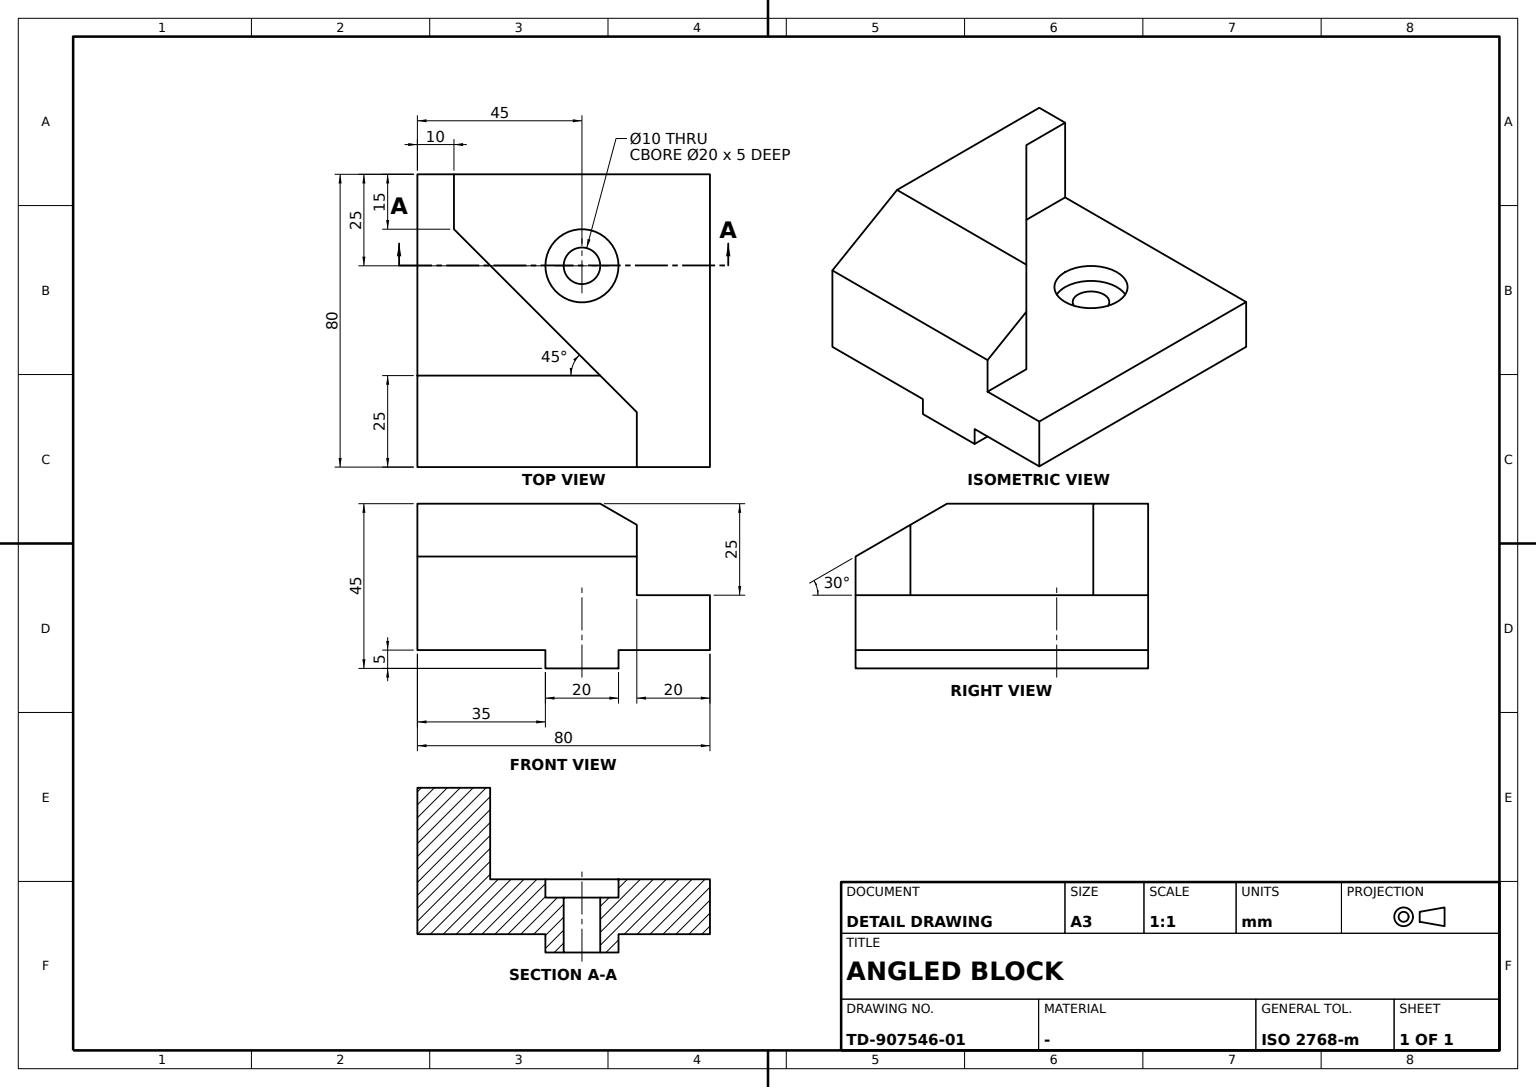
ISO-10303-21;
HEADER;
FILE_DESCRIPTION((''),'2;1');
FILE_NAME('','',(''),(''),'','','');
FILE_SCHEMA(('AUTOMOTIVE_DESIGN'));
ENDSEC;
DATA;
#1=APPLICATION_CONTEXT('');
#2=PRODUCT_CONTEXT('',#1,'mechanical');
#3=PRODUCT('','','',(#2));
#4=PRODUCT_DEFINITION_FORMATION('','',#3);
#5=PRODUCT_DEFINITION_CONTEXT('',#1,'design');
#6=PRODUCT_DEFINITION('','',#4,#5);
#7=PRODUCT_DEFINITION_SHAPE('','',#6);
#8=(LENGTH_UNIT()NAMED_UNIT(*)SI_UNIT(.MILLI.,.METRE.));
#9=(NAMED_UNIT(*)PLANE_ANGLE_UNIT()SI_UNIT($,.RADIAN.));
#10=(NAMED_UNIT(*)SI_UNIT($,.STERADIAN.)SOLID_ANGLE_UNIT());
#11=UNCERTAINTY_MEASURE_WITH_UNIT(LENGTH_MEASURE(0.005),#8,'distance_accuracy_value','');
#12=(GEOMETRIC_REPRESENTATION_CONTEXT(3)GLOBAL_UNCERTAINTY_ASSIGNED_CONTEXT((#11))GLOBAL_UNIT_ASSIGNED_CONTEXT((#8,#9,#10))REPRESENTATION_CONTEXT('',''));
#13=CARTESIAN_POINT('',(50.,15.,-5.));
#14=VERTEX_POINT('',#13);
#15=CARTESIAN_POINT('',(45.,15.,-5.));
#16=DIRECTION('',(0.,0.,1.));
#17=DIRECTION('',(1.,0.,0.));
#18=AXIS2_PLACEMENT_3D('',#15,#16,#17);
#19=CIRCLE('',#18,5.);
#20=EDGE_CURVE('',#14,#14,#19,.T.);
#21=ORIENTED_EDGE('',*,*,#20,.F.);
#22=EDGE_LOOP('',(#21));
#23=FACE_BOUND('',#22,.T.);
#24=CARTESIAN_POINT('',(40.,15.,10.));
#25=VERTEX_POINT('',#24);
#26=CARTESIAN_POINT('',(45.,15.,10.));
#27=DIRECTION('',(0.,0.,-1.));
#28=DIRECTION('',(-1.,0.,0.));
#29=AXIS2_PLACEMENT_3D('',#26,#27,#28);
#30=CIRCLE('',#29,5.);
#31=EDGE_CURVE('',#25,#25,#30,.T.);
#32=ORIENTED_EDGE('',*,*,#31,.F.);
#33=EDGE_LOOP('',(#32));
#34=FACE_BOUND('',#33,.T.);
#35=CARTESIAN_POINT('',(45.,15.,9.9));
#36=AXIS2_PLACEMENT_3D('',#35,#27,#17);
#37=CYLINDRICAL_SURFACE('',#36,5.);
#38=ADVANCED_FACE('',(#23,#34),#37,.F.);
#39=CARTESIAN_POINT('',(55.,40.,0.));
#40=VERTEX_POINT('',#39);
#41=CARTESIAN_POINT('',(55.,-40.,0.));
#42=VERTEX_POINT('',#41);
#43=CARTESIAN_POINT('',(55.,0.,0.));
#44=DIRECTION('',(0.,-1.,0.));
#45=VECTOR('',#44,1000.);
#46=LINE('',#43,#45);
#47=EDGE_CURVE('',#40,#42,#46,.T.);
#48=ORIENTED_EDGE('',*,*,#47,.F.);
#49=CARTESIAN_POINT('',(80.,40.,0.));
#50=VERTEX_POINT('',#49);
#51=VECTOR('',#28,1000.);
#52=LINE('',#49,#51);
#53=EDGE_CURVE('',#50,#40,#52,.T.);
#54=ORIENTED_EDGE('',*,*,#53,.F.);
#55=CARTESIAN_POINT('',(80.,-40.,0.));
#56=VERTEX_POINT('',#55);
#57=CARTESIAN_POINT('',(80.,0.,0.));
#58=LINE('',#57,#45);
#59=EDGE_CURVE('',#50,#56,#58,.T.);
#60=ORIENTED_EDGE('',*,*,#59,.T.);
#61=LINE('',#55,#51);
#62=EDGE_CURVE('',#56,#42,#61,.T.);
#63=ORIENTED_EDGE('',*,*,#62,.T.);
#64=EDGE_LOOP('',(#48,#54,#60,#63));
#65=FACE_BOUND('',#64,.T.);
#66=AXIS2_PLACEMENT_3D('',#57,#16,#28);
#67=PLANE('',#66);
#68=ADVANCED_FACE('',(#65),#67,.F.);
#69=CARTESIAN_POINT('',(60.,-40.,25.566243));
#70=VERTEX_POINT('',#69);
#71=CARTESIAN_POINT('',(60.,-25.,34.226497));
#72=VERTEX_POINT('',#71);
#73=DIRECTION('',(0.,0.866025404,0.5));
#74=VECTOR('',#73,1000.);
#75=LINE('',#69,#74);
#76=EDGE_CURVE('',#70,#72,#75,.T.);
#77=ORIENTED_EDGE('',*,*,#76,.T.);
#78=CARTESIAN_POINT('',(50.,-15.,40.));
#79=VERTEX_POINT('',#78);
#80=CARTESIAN_POINT('',(21.900181,13.099819,56.223438));
#81=DIRECTION('',(0.654653671,-0.654653671,-0.377964473));
#82=VECTOR('',#81,1000.);
#83=LINE('',#80,#82);
#84=EDGE_CURVE('',#79,#72,#83,.T.);
#85=ORIENTED_EDGE('',*,*,#84,.F.);
#86=CARTESIAN_POINT('',(0.,-15.,40.));
#87=VERTEX_POINT('',#86);
#88=VECTOR('',#17,1000.);
#89=LINE('',#86,#88);
#90=EDGE_CURVE('',#87,#79,#89,.T.);
#91=ORIENTED_EDGE('',*,*,#90,.F.);
#92=CARTESIAN_POINT('',(0.,-40.,25.566243));
#93=VERTEX_POINT('',#92);
#94=CARTESIAN_POINT('',(0.,-21.070508,36.495191));
#95=LINE('',#94,#74);
#96=EDGE_CURVE('',#93,#87,#95,.T.);
#97=ORIENTED_EDGE('',*,*,#96,.F.);
#98=LINE('',#92,#88);
#99=EDGE_CURVE('',#93,#70,#98,.T.);
#100=ORIENTED_EDGE('',*,*,#99,.T.);
#101=EDGE_LOOP('',(#77,#85,#91,#97,#100));
#102=FACE_BOUND('',#101,.T.);
#103=DIRECTION('',(0.,0.5,-0.866025404));
#104=AXIS2_PLACEMENT_3D('',#92,#103,#73);
#105=PLANE('',#104);
#106=ADVANCED_FACE('',(#102),#105,.F.);
#107=CARTESIAN_POINT('',(55.,40.,-5.));
#108=VERTEX_POINT('',#107);
#109=VECTOR('',#27,1000.);
#110=LINE('',#39,#109);
#111=EDGE_CURVE('',#40,#108,#110,.T.);
#112=ORIENTED_EDGE('',*,*,#111,.F.);
#113=ORIENTED_EDGE('',*,*,#47,.T.);
#114=CARTESIAN_POINT('',(55.,-40.,-5.));
#115=VERTEX_POINT('',#114);
#116=LINE('',#41,#109);
#117=EDGE_CURVE('',#42,#115,#116,.T.);
#118=ORIENTED_EDGE('',*,*,#117,.T.);
#119=CARTESIAN_POINT('',(55.,0.,-5.));
#120=LINE('',#119,#45);
#121=EDGE_CURVE('',#108,#115,#120,.T.);
#122=ORIENTED_EDGE('',*,*,#121,.F.);
#123=EDGE_LOOP('',(#112,#113,#118,#122));
#124=FACE_BOUND('',#123,.T.);
#125=AXIS2_PLACEMENT_3D('',#43,#28,#27);
#126=PLANE('',#125);
#127=ADVANCED_FACE('',(#124),#126,.F.);
#128=ORIENTED_EDGE('',*,*,#84,.T.);
#129=CARTESIAN_POINT('',(60.,-25.,15.));
#130=VERTEX_POINT('',#129);
#131=LINE('',#129,#109);
#132=EDGE_CURVE('',#72,#130,#131,.T.);
#133=ORIENTED_EDGE('',*,*,#132,.T.);
#134=CARTESIAN_POINT('',(10.,25.,15.));
#135=VERTEX_POINT('',#134);
#136=DIRECTION('',(0.707106781,-0.707106781,0.));
#137=VECTOR('',#136,1000.);
#138=LINE('',#134,#137);
#139=EDGE_CURVE('',#135,#130,#138,.T.);
#140=ORIENTED_EDGE('',*,*,#139,.F.);
#141=CARTESIAN_POINT('',(10.,25.,40.));
#142=VERTEX_POINT('',#141);
#143=VECTOR('',#16,1000.);
#144=LINE('',#141,#143);
#145=EDGE_CURVE('',#135,#142,#144,.T.);
#146=ORIENTED_EDGE('',*,*,#145,.T.);
#147=LINE('',#141,#137);
#148=EDGE_CURVE('',#142,#79,#147,.T.);
#149=ORIENTED_EDGE('',*,*,#148,.T.);
#150=EDGE_LOOP('',(#128,#133,#140,#146,#149));
#151=FACE_BOUND('',#150,.T.);
#152=DIRECTION('',(-0.707106781,-0.707106781,0.));
#153=AXIS2_PLACEMENT_3D('',#134,#152,#136);
#154=PLANE('',#153);
#155=ADVANCED_FACE('',(#151),#154,.F.);
#156=CARTESIAN_POINT('',(35.,40.,-5.));
#157=VERTEX_POINT('',#156);
#158=CARTESIAN_POINT('',(35.,40.,0.));
#159=VERTEX_POINT('',#158);
#160=LINE('',#156,#143);
#161=EDGE_CURVE('',#157,#159,#160,.T.);
#162=ORIENTED_EDGE('',*,*,#161,.T.);
#163=CARTESIAN_POINT('',(0.,40.,0.));
#164=VERTEX_POINT('',#163);
#165=EDGE_CURVE('',#159,#164,#52,.T.);
#166=ORIENTED_EDGE('',*,*,#165,.T.);
#167=CARTESIAN_POINT('',(0.,40.,40.));
#168=VERTEX_POINT('',#167);
#169=LINE('',#163,#143);
#170=EDGE_CURVE('',#164,#168,#169,.T.);
#171=ORIENTED_EDGE('',*,*,#170,.T.);
#172=CARTESIAN_POINT('',(10.,40.,40.));
#173=VERTEX_POINT('',#172);
#174=LINE('',#167,#88);
#175=EDGE_CURVE('',#168,#173,#174,.T.);
#176=ORIENTED_EDGE('',*,*,#175,.T.);
#177=CARTESIAN_POINT('',(10.,40.,15.));
#178=VERTEX_POINT('',#177);
#179=LINE('',#172,#109);
#180=EDGE_CURVE('',#173,#178,#179,.T.);
#181=ORIENTED_EDGE('',*,*,#180,.T.);
#182=CARTESIAN_POINT('',(80.,40.,15.));
#183=VERTEX_POINT('',#182);
#184=LINE('',#177,#88);
#185=EDGE_CURVE('',#178,#183,#184,.T.);
#186=ORIENTED_EDGE('',*,*,#185,.T.);
#187=LINE('',#182,#109);
#188=EDGE_CURVE('',#183,#50,#187,.T.);
#189=ORIENTED_EDGE('',*,*,#188,.T.);
#190=ORIENTED_EDGE('',*,*,#53,.T.);
#191=ORIENTED_EDGE('',*,*,#111,.T.);
#192=LINE('',#107,#51);
#193=EDGE_CURVE('',#108,#157,#192,.T.);
#194=ORIENTED_EDGE('',*,*,#193,.T.);
#195=EDGE_LOOP('',(#162,#166,#171,#176,#181,#186,#189,#190,#191,#194));
#196=FACE_BOUND('',#195,.T.);
#197=DIRECTION('',(0.,1.,0.));
#198=AXIS2_PLACEMENT_3D('',#163,#197,#28);
#199=PLANE('',#198);
#200=ADVANCED_FACE('',(#196),#199,.T.);
#201=CARTESIAN_POINT('',(0.,0.,40.));
#202=LINE('',#201,#45);
#203=EDGE_CURVE('',#168,#87,#202,.T.);
#204=ORIENTED_EDGE('',*,*,#203,.T.);
#205=ORIENTED_EDGE('',*,*,#90,.T.);
#206=ORIENTED_EDGE('',*,*,#148,.F.);
#207=CARTESIAN_POINT('',(10.,0.,40.));
#208=LINE('',#207,#45);
#209=EDGE_CURVE('',#173,#142,#208,.T.);
#210=ORIENTED_EDGE('',*,*,#209,.F.);
#211=ORIENTED_EDGE('',*,*,#175,.F.);
#212=EDGE_LOOP('',(#204,#205,#206,#210,#211));
#213=FACE_BOUND('',#212,.T.);
#214=AXIS2_PLACEMENT_3D('',#201,#27,#17);
#215=PLANE('',#214);
#216=ADVANCED_FACE('',(#213),#215,.F.);
#217=CARTESIAN_POINT('',(35.,15.,10.));
#218=VERTEX_POINT('',#217);
#219=CIRCLE('',#29,10.);
#220=EDGE_CURVE('',#218,#218,#219,.T.);
#221=ORIENTED_EDGE('',*,*,#220,.T.);
#222=EDGE_LOOP('',(#221));
#223=FACE_BOUND('',#222,.T.);
#224=CARTESIAN_POINT('',(35.,15.,15.));
#225=VERTEX_POINT('',#224);
#226=CARTESIAN_POINT('',(45.,15.,15.));
#227=AXIS2_PLACEMENT_3D('',#226,#27,#28);
#228=CIRCLE('',#227,10.);
#229=EDGE_CURVE('',#225,#225,#228,.T.);
#230=ORIENTED_EDGE('',*,*,#229,.F.);
#231=EDGE_LOOP('',(#230));
#232=FACE_BOUND('',#231,.T.);
#233=CARTESIAN_POINT('',(45.,15.,14.9));
#234=AXIS2_PLACEMENT_3D('',#233,#27,#17);
#235=CYLINDRICAL_SURFACE('',#234,10.);
#236=ADVANCED_FACE('',(#223,#232),#235,.F.);
#237=ORIENTED_EDGE('',*,*,#203,.F.);
#238=ORIENTED_EDGE('',*,*,#170,.F.);
#239=CARTESIAN_POINT('',(0.,-40.,0.));
#240=VERTEX_POINT('',#239);
#241=CARTESIAN_POINT('',(0.,0.,0.));
#242=LINE('',#241,#45);
#243=EDGE_CURVE('',#164,#240,#242,.T.);
#244=ORIENTED_EDGE('',*,*,#243,.T.);
#245=LINE('',#239,#143);
#246=EDGE_CURVE('',#240,#93,#245,.T.);
#247=ORIENTED_EDGE('',*,*,#246,.T.);
#248=ORIENTED_EDGE('',*,*,#96,.T.);
#249=EDGE_LOOP('',(#237,#238,#244,#247,#248));
#250=FACE_BOUND('',#249,.T.);
#251=AXIS2_PLACEMENT_3D('',#241,#17,#16);
#252=PLANE('',#251);
#253=ADVANCED_FACE('',(#250),#252,.F.);
#254=CARTESIAN_POINT('',(80.,-40.,15.));
#255=VERTEX_POINT('',#254);
#256=LINE('',#254,#109);
#257=EDGE_CURVE('',#255,#56,#256,.T.);
#258=ORIENTED_EDGE('',*,*,#257,.T.);
#259=ORIENTED_EDGE('',*,*,#59,.F.);
#260=ORIENTED_EDGE('',*,*,#188,.F.);
#261=CARTESIAN_POINT('',(80.,0.,15.));
#262=LINE('',#261,#45);
#263=EDGE_CURVE('',#183,#255,#262,.T.);
#264=ORIENTED_EDGE('',*,*,#263,.T.);
#265=EDGE_LOOP('',(#258,#259,#260,#264));
#266=FACE_BOUND('',#265,.T.);
#267=AXIS2_PLACEMENT_3D('',#261,#28,#27);
#268=PLANE('',#267);
#269=ADVANCED_FACE('',(#266),#268,.F.);
#270=ORIENTED_EDGE('',*,*,#145,.F.);
#271=CARTESIAN_POINT('',(10.,0.,15.));
#272=LINE('',#271,#45);
#273=EDGE_CURVE('',#178,#135,#272,.T.);
#274=ORIENTED_EDGE('',*,*,#273,.F.);
#275=ORIENTED_EDGE('',*,*,#180,.F.);
#276=ORIENTED_EDGE('',*,*,#209,.T.);
#277=EDGE_LOOP('',(#270,#274,#275,#276));
#278=FACE_BOUND('',#277,.T.);
#279=AXIS2_PLACEMENT_3D('',#207,#28,#27);
#280=PLANE('',#279);
#281=ADVANCED_FACE('',(#278),#280,.F.);
#282=ORIENTED_EDGE('',*,*,#229,.T.);
#283=EDGE_LOOP('',(#282));
#284=FACE_BOUND('',#283,.T.);
#285=ORIENTED_EDGE('',*,*,#185,.F.);
#286=ORIENTED_EDGE('',*,*,#273,.T.);
#287=ORIENTED_EDGE('',*,*,#139,.T.);
#288=CARTESIAN_POINT('',(60.,-40.,15.));
#289=VERTEX_POINT('',#288);
#290=CARTESIAN_POINT('',(60.,0.,15.));
#291=VECTOR('',#197,1000.);
#292=LINE('',#290,#291);
#293=EDGE_CURVE('',#289,#130,#292,.T.);
#294=ORIENTED_EDGE('',*,*,#293,.F.);
#295=CARTESIAN_POINT('',(0.,-40.,15.));
#296=LINE('',#295,#51);
#297=EDGE_CURVE('',#255,#289,#296,.T.);
#298=ORIENTED_EDGE('',*,*,#297,.F.);
#299=ORIENTED_EDGE('',*,*,#263,.F.);
#300=EDGE_LOOP('',(#285,#286,#287,#294,#298,#299));
#301=FACE_BOUND('',#300,.T.);
#302=AXIS2_PLACEMENT_3D('',#271,#27,#17);
#303=PLANE('',#302);
#304=ADVANCED_FACE('',(#284,#301),#303,.F.);
#305=ORIENTED_EDGE('',*,*,#297,.T.);
#306=CARTESIAN_POINT('',(60.,-40.,40.));
#307=LINE('',#306,#109);
#308=EDGE_CURVE('',#70,#289,#307,.T.);
#309=ORIENTED_EDGE('',*,*,#308,.F.);
#310=ORIENTED_EDGE('',*,*,#99,.F.);
#311=ORIENTED_EDGE('',*,*,#246,.F.);
#312=CARTESIAN_POINT('',(35.,-40.,0.));
#313=VERTEX_POINT('',#312);
#314=EDGE_CURVE('',#313,#240,#61,.T.);
#315=ORIENTED_EDGE('',*,*,#314,.F.);
#316=CARTESIAN_POINT('',(35.,-40.,-5.));
#317=VERTEX_POINT('',#316);
#318=LINE('',#316,#143);
#319=EDGE_CURVE('',#317,#313,#318,.T.);
#320=ORIENTED_EDGE('',*,*,#319,.F.);
#321=LINE('',#114,#51);
#322=EDGE_CURVE('',#115,#317,#321,.T.);
#323=ORIENTED_EDGE('',*,*,#322,.F.);
#324=ORIENTED_EDGE('',*,*,#117,.F.);
#325=ORIENTED_EDGE('',*,*,#62,.F.);
#326=ORIENTED_EDGE('',*,*,#257,.F.);
#327=EDGE_LOOP('',(#305,#309,#310,#311,#315,#320,#323,#324,#325,#326));
#328=FACE_BOUND('',#327,.T.);
#329=AXIS2_PLACEMENT_3D('',#239,#197,#28);
#330=PLANE('',#329);
#331=ADVANCED_FACE('',(#328),#330,.F.);
#332=ORIENTED_EDGE('',*,*,#314,.T.);
#333=ORIENTED_EDGE('',*,*,#243,.F.);
#334=ORIENTED_EDGE('',*,*,#165,.F.);
#335=CARTESIAN_POINT('',(35.,0.,0.));
#336=LINE('',#335,#45);
#337=EDGE_CURVE('',#159,#313,#336,.T.);
#338=ORIENTED_EDGE('',*,*,#337,.T.);
#339=EDGE_LOOP('',(#332,#333,#334,#338));
#340=FACE_BOUND('',#339,.T.);
#341=ADVANCED_FACE('',(#340),#67,.F.);
#342=ORIENTED_EDGE('',*,*,#193,.F.);
#343=ORIENTED_EDGE('',*,*,#121,.T.);
#344=ORIENTED_EDGE('',*,*,#322,.T.);
#345=CARTESIAN_POINT('',(35.,0.,-5.));
#346=LINE('',#345,#45);
#347=EDGE_CURVE('',#157,#317,#346,.T.);
#348=ORIENTED_EDGE('',*,*,#347,.F.);
#349=EDGE_LOOP('',(#342,#343,#344,#348));
#350=FACE_BOUND('',#349,.T.);
#351=ORIENTED_EDGE('',*,*,#20,.T.);
#352=EDGE_LOOP('',(#351));
#353=FACE_BOUND('',#352,.T.);
#354=AXIS2_PLACEMENT_3D('',#119,#16,#28);
#355=PLANE('',#354);
#356=ADVANCED_FACE('',(#350,#353),#355,.F.);
#357=ORIENTED_EDGE('',*,*,#220,.F.);
#358=EDGE_LOOP('',(#357));
#359=FACE_BOUND('',#358,.T.);
#360=ORIENTED_EDGE('',*,*,#31,.T.);
#361=EDGE_LOOP('',(#360));
#362=FACE_BOUND('',#361,.T.);
#363=AXIS2_PLACEMENT_3D('',#26,#27,#17);
#364=PLANE('',#363);
#365=ADVANCED_FACE('',(#359,#362),#364,.F.);
#366=ORIENTED_EDGE('',*,*,#76,.F.);
#367=ORIENTED_EDGE('',*,*,#308,.T.);
#368=ORIENTED_EDGE('',*,*,#293,.T.);
#369=ORIENTED_EDGE('',*,*,#132,.F.);
#370=EDGE_LOOP('',(#366,#367,#368,#369));
#371=FACE_BOUND('',#370,.T.);
#372=AXIS2_PLACEMENT_3D('',#306,#28,#197);
#373=PLANE('',#372);
#374=ADVANCED_FACE('',(#371),#373,.F.);
#375=ORIENTED_EDGE('',*,*,#347,.T.);
#376=ORIENTED_EDGE('',*,*,#319,.T.);
#377=ORIENTED_EDGE('',*,*,#337,.F.);
#378=ORIENTED_EDGE('',*,*,#161,.F.);
#379=EDGE_LOOP('',(#375,#376,#377,#378));
#380=FACE_BOUND('',#379,.T.);
#381=AXIS2_PLACEMENT_3D('',#345,#17,#16);
#382=PLANE('',#381);
#383=ADVANCED_FACE('',(#380),#382,.F.);
#384=CLOSED_SHELL('',(#38,#68,#106,#127,#155,#200,#216,#236,#253,#269,#281,#304,#331,#341,#356,#365,#374,#383));
#385=MANIFOLD_SOLID_BREP('',#384);
#386=ADVANCED_BREP_SHAPE_REPRESENTATION('',(#385),#12);
#387=SHAPE_DEFINITION_REPRESENTATION(#7,#386);
ENDSEC;
END-ISO-10303-21;
